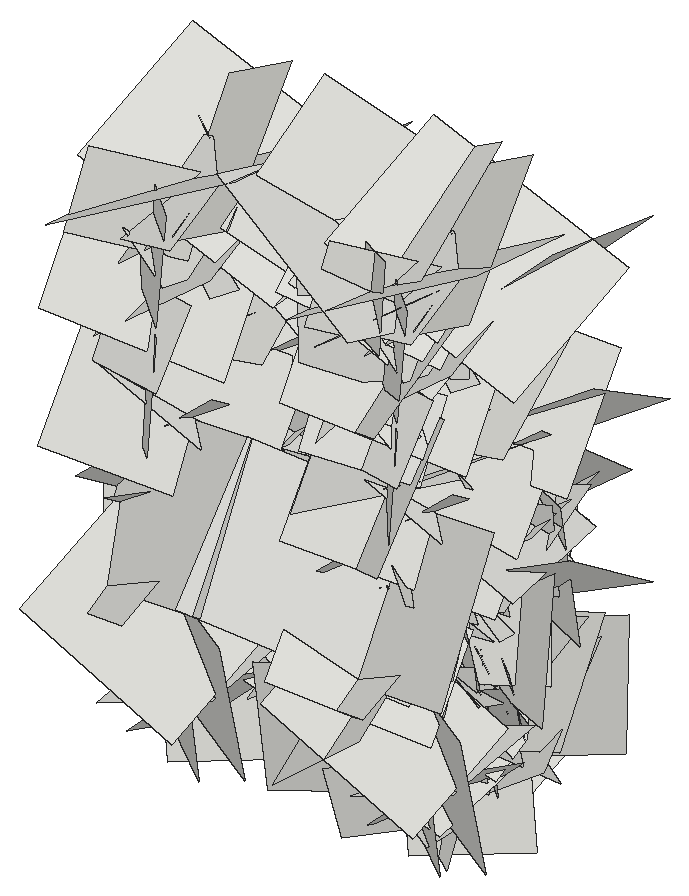
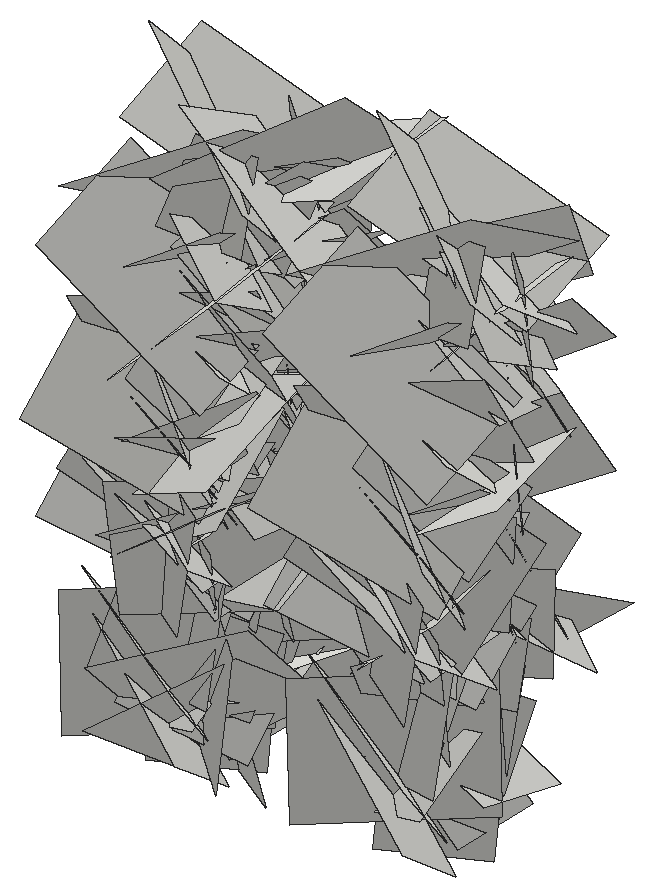
# SketchUp Ruby script. Lengths in inches.
U = 1.inch
M = Sketchup.active_model
def pt(a) = Geom::Point3d.new(a.map { |v| v * U })
def face(e, loops, mat)
  f = e.add_face(loops[0].map { |a| pt(a) })
  loops[1..].each { |l| e.add_face(l.map { |a| pt(a) }).erase! }
  f.material = f.back_material = mat if mat
  f
end
# faces: each face lists its corners as indices into pts; further lists are holes
def faces(e, pts, list, mat = nil) = list.each { |f| face(e, (f[0].is_a?(Array) ? f : [f]).map { |l| l.map { |i| pts[i] } }, mat) }
# xy, xz, yz: faces in a plane at the given z, y or x. An outline is a flat list of corners, or four numbers for a rectangle; further outlines are holes
def ring(l) = l.size == 4 ? [[l[0], l[1]], [l[2], l[1]], [l[2], l[3]], [l[0], l[3]]] : l.each_slice(2).to_a
def flat(e, list, mat, &to3) = list.each { |f| face(e, (f[0].is_a?(Array) ? f : [f]).map { |l| ring(l).map { |u, v| to3.(u, v) } }, mat) }
def xy(e, z, list, mat = nil) = flat(e, list, mat) { |x, y| [x, y, z] }
def xz(e, y, list, mat = nil) = flat(e, list, mat) { |x, z| [x, y, z] }
def yz(e, x, list, mat = nil) = flat(e, list, mat) { |y, z| [x, y, z] }
def lines(e, pts, list) = list.each { |a, b| e.add_line(pt(pts[a]), pt(pts[b])) }
# prism: a flat outline (further loops are holes) pulled along v
def prism(e, loops, v, mat = nil)
  f = face(e, loops, mat); d = Geom::Vector3d.new(v.map { |x| x * U })
  f.pushpull(f.normal.samedirection?(d) ? d.length : -d.length)
end
def box(e, o, s, mat = nil) = prism(e, [[o, [o[0] + s[0], o[1], o[2]], [o[0] + s[0], o[1] + s[1], o[2]], [o[0], o[1] + s[1], o[2]]]], [0, 0, s[2]], mat)
def at(x, y, z, deg = 0) = Geom::Transformation.translation(pt([x, y, z])) * Geom::Transformation.rotation(ORIGIN, Z_AXIS, deg.degrees)
def axes(o, x, y, z) = Geom::Transformation.new([*x, 0, *y, 0, *z, 0, *pt(o).to_a, 1])
def part(name) = M.definitions.add(name)
# library, detail: a bought-in or finely detailed component or shape, given as its bounding box
def library(name, o, s) = part(name).tap { |d| box(d.entities, o, s) }
def detail(e, o, s) = box(e.add_group.entities, o, s)
def put(e, d, t, mat = nil) = e.add_instance(d, t).tap { |i| i.material = mat if mat }
def group(e, t, mat = nil) = e.add_group.tap { |g| g.transformation = t; g.material = mat if mat }.entities
root = M.entities
c1 = part("Component\#6")
p = [[0.01,0,0],[0,3.24,4.54],[4.32,3.24,4.54],[4.33,0,0]]
faces(c1.entities,p,[[0,1,2,3]])
put(root,c1,axes([410.71,170.9375,7.01],[0.11124,0.9843,0.53665],[-0.15751,0.54645,-0.97322],[1.17787,-0.01989,-0.18083]))
put(root,c1,axes([424.49,170.9375,7.01],[-0.11124,0.9843,0.53665],[0.15751,0.54645,-0.97322],[-1.17787,-0.01989,-0.18083]))
put(root,c1,axes([420.52,170.9375,7.01],[0.11124,0.9843,0.53665],[-0.15751,0.54645,-0.97322],[1.17787,-0.01989,-0.18083]))
put(root,c1,axes([410.71,177.17,11.87],[0.09089,-0.73345,-1.16692],[0.11565,-1.16189,0.73831],[1.45639,0.13804,0.0142]))
put(root,c1,axes([424.49,177.17,11.87],[-0.09089,-0.73345,-1.16692],[-0.11565,-1.16189,0.73831],[-1.45639,0.13804,0.0142]))
put(root,c1,axes([420.52,177.17,11.87],[0.09089,-0.73345,-1.16692],[0.11565,-1.16189,0.73831],[1.45639,0.13804,0.0142]))
put(root,c1,axes([414.68,171.15,7.72],[0.19789,0.75168,0.59634],[-0.00491,0.60823,-0.76521],[-1.01706,0.14332,0.11972]))
put(root,c1,axes([420.52,171.15,7.72],[-0.19789,0.75168,0.59634],[0.00491,0.60823,-0.76521],[1.01706,0.14332,0.11972]))
put(root,c1,axes([424.49,171.15,7.72],[0.19789,0.75168,0.59634],[-0.00491,0.60823,-0.76521],[-1.01706,0.14332,0.11972]))
put(root,c1,axes([414.68,175.79,22.11],[-0.09057,-0.18477,-0.67682],[0.07729,-0.68047,0.17656],[-0.73966,-0.04848,0.10132]))
put(root,c1,axes([420.52,175.79,22.11],[0.09057,-0.18477,-0.67682],[-0.07729,-0.68047,0.17656],[0.73966,-0.04848,0.10132]))
put(root,c1,axes([424.49,175.79,22.11],[-0.09057,-0.18477,-0.67682],[0.07729,-0.68047,0.17656],[-0.73966,-0.04848,0.10132]))
put(root,c1,axes([414.68,172.87,15.39],[0.04258,0.36909,0.59744],[-0.18529,0.58484,-0.34955],[-0.72096,-0.1285,0.12512]))
put(root,c1,axes([420.52,172.87,15.39],[-0.04258,0.36909,0.59744],[0.18529,0.58484,-0.34955],[0.72096,-0.1285,0.12512]))
put(root,c1,axes([424.49,172.87,15.39],[0.04258,0.36909,0.59744],[-0.18529,0.58484,-0.34955],[-0.72096,-0.1285,0.12512]))
put(root,c1,axes([410.71,176.71,20],[0.1716,-1.2405,0.25629],[0.15029,0.2745,1.23906],[1.33426,0.12862,-0.17253]))
put(root,c1,axes([424.49,176.71,20],[-0.1716,-1.2405,0.25629],[-0.15029,0.2745,1.23906],[-1.33426,0.12862,-0.17253]))
put(root,c1,axes([420.52,176.71,20],[0.1716,-1.2405,0.25629],[0.15029,0.2745,1.23906],[1.33426,0.12862,-0.17253]))
put(root,c1,axes([414.68,172.9,17.79],[0.05847,0.04666,0.93522],[0.13105,0.92828,-0.05361],[-0.98388,0.12642,0.04844]))
put(root,c1,axes([420.52,172.9,17.79],[-0.05847,0.04666,0.93522],[-0.13105,0.92828,-0.05361],[0.98388,0.12642,0.04844]))
put(root,c1,axes([424.49,172.9,17.79],[0.05847,0.04666,0.93522],[0.13105,0.92828,-0.05361],[-0.98388,0.12642,0.04844]))
put(root,c1,axes([414.68,172.44,13.26],[-0.14239,0.27787,0.83247],[0.25689,0.82117,-0.23499],[-0.89411,0.19168,-0.20009]))
put(root,c1,axes([420.52,172.44,13.26],[0.14239,0.27787,0.83247],[-0.25689,0.82117,-0.23499],[0.89411,0.19168,-0.20009]))
put(root,c1,axes([424.49,172.44,13.26],[-0.14239,0.27787,0.83247],[0.25689,0.82117,-0.23499],[-0.89411,0.19168,-0.20009]))
put(root,c1,axes([414.68,178.76,18.36],[0.19902,-0.79911,-0.76231],[0.1591,-0.74761,0.82067],[-1.1598,-0.23968,-0.01823]))
put(root,c1,axes([420.52,178.76,18.36],[-0.19902,-0.79911,-0.76231],[-0.1591,-0.74761,0.82067],[1.1598,-0.23968,-0.01823]))
put(root,c1,axes([424.49,178.76,18.36],[0.19902,-0.79911,-0.76231],[0.1591,-0.74761,0.82067],[-1.1598,-0.23968,-0.01823]))
put(root,c1,axes([410.71,178.02,21.625],[-0.10055,-0.80704,-0.57155],[0.14009,-0.57937,0.79615],[1.03886,0.00001,-0.16268]))
put(root,c1,axes([424.49,178.02,21.625],[0.10055,-0.80704,-0.57155],[-0.14009,-0.57937,0.79615],[-1.03886,0.00001,-0.16268]))
put(root,c1,axes([420.52,178.02,21.625],[-0.10055,-0.80704,-0.57155],[0.14009,-0.57937,0.79615],[1.03886,0.00001,-0.16268]))
put(root,c1,axes([410.71,171.875,12.53],[-0.03767,0.74177,1.03266],[-0.14299,1.02503,-0.74093],[1.34014,0.13022,-0.05004]))
put(root,c1,axes([424.49,171.875,12.53],[0.03767,0.74177,1.03266],[0.14299,1.02503,-0.74093],[-1.34014,0.13022,-0.05004]))
put(root,c1,axes([420.52,171.875,12.53],[-0.03767,0.74177,1.03266],[-0.14299,1.02503,-0.74093],[1.34014,0.13022,-0.05004]))
put(root,c1,axes([414.68,176.92,18.36],[-0.03591,-0.7978,0.13647],[0.05211,0.13431,0.79737],[-0.85636,0.04162,0.0428]))
put(root,c1,axes([420.52,176.92,18.36],[0.03591,-0.7978,0.13647],[-0.05211,0.13431,0.79737],[0.85636,0.04162,0.0428]))
put(root,c1,axes([424.49,176.92,18.36],[-0.03591,-0.7978,0.13647],[0.05211,0.13431,0.79737],[-0.85636,0.04162,0.0428]))
put(root,c1,axes([410.71,176.79,7.17],[0.05072,0.23896,-1.1979],[0.10512,-1.19562,-0.23454],[1.29052,0.088,0.06618]))
put(root,c1,axes([424.49,176.79,7.17],[-0.05072,0.23896,-1.1979],[-0.10512,-1.19562,-0.23454],[-1.29052,0.088,0.06618]))
put(root,c1,axes([420.52,176.79,7.17],[0.05072,0.23896,-1.1979],[0.10512,-1.19562,-0.23454],[1.29052,0.088,0.06618]))
put(root,c1,axes([414.68,175.07,0.3],[0.05353,-0.16234,0.63718],[0.01427,0.63917,0.16178],[-0.69684,0.00062,0.05226]))
put(root,c1,axes([420.52,175.07,0.3],[-0.05353,-0.16234,0.63718],[-0.01427,0.63917,0.16178],[0.69684,0.00062,0.05226]))
put(root,c1,axes([424.49,175.07,0.3],[0.05353,-0.16234,0.63718],[0.01427,0.63917,0.16178],[-0.69684,0.00062,0.05226]))
put(root,c1,axes([410.71,178.16,17.01],[0.17232,-1.0163,-0.23365],[-0.0611,-0.24487,1.02499],[1.10369,0.14512,0.09322]))
put(root,c1,axes([424.49,178.16,17.01],[-0.17232,-1.0163,-0.23365],[0.0611,-0.24487,1.02499],[-1.10369,0.14512,0.09322]))
put(root,c1,axes([420.52,178.16,17.01],[0.17232,-1.0163,-0.23365],[-0.0611,-0.24487,1.02499],[1.10369,0.14512,0.09322]))
put(root,c1,axes([410.71,178.75,19.8],[0.0392,-0.90326,-0.49419],[-0.16181,-0.49385,0.89122],[1.07932,-0.04123,0.15156]))
put(root,c1,axes([424.49,178.75,19.8],[-0.0392,-0.90326,-0.49419],[0.16181,-0.49385,0.89122],[-1.07932,-0.04123,0.15156]))
put(root,c1,axes([420.52,178.75,19.8],[0.0392,-0.90326,-0.49419],[-0.16181,-0.49385,0.89122],[1.07932,-0.04123,0.15156]))
put(root,c1,axes([414.68,174.43,8.39],[0.03188,0.26889,0.69876],[-0.00311,0.69936,-0.269],[-0.79363,0.00806,0.02912]))
put(root,c1,axes([420.52,174.43,8.39],[-0.03188,0.26889,0.69876],[0.00311,0.69936,-0.269],[0.79363,0.00806,0.02912]))
put(root,c1,axes([424.49,174.43,8.39],[0.03188,0.26889,0.69876],[-0.00311,0.69936,-0.269],[-0.79363,0.00806,0.02912]))
put(root,c1,axes([410.71,179.79,22.45],[0.18749,-0.99323,-0.93091],[-0.09936,-0.94539,0.99088],[1.43954,0.06411,0.18963]))
put(root,c1,axes([424.49,179.79,22.45],[-0.18749,-0.99323,-0.93091],[0.09936,-0.94539,0.99088],[-1.43954,0.06411,0.18963]))
put(root,c1,axes([420.52,179.79,22.45],[0.18749,-0.99323,-0.93091],[-0.09936,-0.94539,0.99088],[1.43954,0.06411,0.18963]))
put(root,c1,axes([410.71,177.03,8.61],[0.03763,-0.79919,0.49947],[-0.19388,0.48448,0.78821],[0.97999,0.12653,0.13676]))
put(root,c1,axes([424.49,177.03,8.61],[-0.03763,-0.79919,0.49947],[0.19388,0.48448,0.78821],[-0.97999,0.12653,0.13676]))
put(root,c1,axes([420.52,177.03,8.61],[0.03763,-0.79919,0.49947],[-0.19388,0.48448,0.78821],[0.97999,0.12653,0.13676]))
put(root,c1,axes([414.68,177.03,9.04],[0.05145,-0.49737,0.47013],[-0.11624,0.45957,0.49752],[-0.71609,-0.11034,-0.04698]))
put(root,c1,axes([420.52,177.03,9.04],[-0.05145,-0.49737,0.47013],[0.11624,0.45957,0.49752],[0.71609,-0.11034,-0.04698]))
put(root,c1,axes([424.49,177.03,9.04],[0.05145,-0.49737,0.47013],[-0.11624,0.45957,0.49752],[-0.71609,-0.11034,-0.04698]))
put(root,c1,axes([410.71,179.02,2.63],[-0.02304,-0.93672,-0.18796],[0.20199,-0.18848,0.91728],[0.99236,0.01662,-0.19107]))
put(root,c1,axes([424.49,179.02,2.63],[0.02304,-0.93672,-0.18796],[-0.20199,-0.18848,0.91728],[-0.99236,0.01662,-0.19107]))
put(root,c1,axes([420.52,179.02,2.63],[-0.02304,-0.93672,-0.18796],[0.20199,-0.18848,0.91728],[0.99236,0.01662,-0.19107]))
put(root,c1,axes([414.68,175.31,3.87],[0.17194,0.72285,-0.14796],[0.1038,-0.17124,-0.72925],[-0.77519,0.1374,-0.13047]))
put(root,c1,axes([420.52,175.31,3.87],[-0.17194,0.72285,-0.14796],[-0.1038,-0.17124,-0.72925],[0.77519,0.1374,-0.13047]))
put(root,c1,axes([424.49,175.31,3.87],[0.17194,0.72285,-0.14796],[0.1038,-0.17124,-0.72925],[-0.77519,0.1374,-0.13047]))
put(root,c1,axes([410.71,173.88,22.27],[0.13701,1.18016,0.66561],[0.07419,0.66193,-1.18721],[1.4343,-0.14697,-0.00217]))
put(root,c1,axes([424.49,173.88,22.27],[-0.13701,1.18016,0.66561],[-0.07419,0.66193,-1.18721],[-1.4343,-0.14697,-0.00217]))
put(root,c1,axes([420.52,173.88,22.27],[0.13701,1.18016,0.66561],[0.07419,0.66193,-1.18721],[1.4343,-0.14697,-0.00217]))
put(root,c1,axes([410.71,175.28,5.97],[-0.1544,0.17587,1.10387],[0.02973,1.11343,-0.17369],[1.18449,-0.00502,0.14825]))
put(root,c1,axes([424.49,175.28,5.97],[0.1544,0.17587,1.10387],[-0.02973,1.11343,-0.17369],[-1.18449,-0.00502,0.14825]))
put(root,c1,axes([420.52,175.28,5.97],[-0.1544,0.17587,1.10387],[0.02973,1.11343,-0.17369],[1.18449,-0.00502,0.14825]))
put(root,c1,axes([410.71,174.05,15.13],[-0.29087,1.34123,-0.04275],[0.1118,-0.02194,-1.36543],[1.41802,0.27684,0.09888]))
put(root,c1,axes([424.49,174.05,15.13],[0.29087,1.34123,-0.04275],[-0.1118,-0.02194,-1.36543],[-1.41802,0.27684,0.09888]))
put(root,c1,axes([420.52,174.05,15.13],[-0.29087,1.34123,-0.04275],[0.1118,-0.02194,-1.36543],[1.41802,0.27684,0.09888]))
put(root,c1,axes([410.71,177.91,2.6],[0.0759,-0.493,0.60539],[0.11612,0.60826,0.48238],[0.8194,-0.04053,-0.12444]))
put(root,c1,axes([424.49,177.91,2.6],[-0.0759,-0.493,0.60539],[-0.11612,0.60826,0.48238],[-0.8194,-0.04053,-0.12444]))
put(root,c1,axes([420.52,177.91,2.6],[0.0759,-0.493,0.60539],[0.11612,0.60826,0.48238],[0.8194,-0.04053,-0.12444]))
put(root,c1,axes([414.68,179.07,16.9375],[-0.01654,-0.76992,0.15337],[0.18248,0.14631,0.752],[-0.8119,0.04857,0.16589]))
put(root,c1,axes([420.52,179.07,16.9375],[0.01654,-0.76992,0.15337],[-0.18248,0.14631,0.752],[0.8119,0.04857,0.16589]))
put(root,c1,axes([424.49,179.07,16.9375],[-0.01654,-0.76992,0.15337],[0.18248,0.14631,0.752],[-0.8119,0.04857,0.16589]))
put(root,c1,axes([410.71,177.25,5.58],[0.00826,-0.19404,0.73725],[0.12542,0.72866,0.19053],[0.79831,-0.11247,-0.03756]))
put(root,c1,axes([424.49,177.25,5.58],[-0.00826,-0.19404,0.73725],[-0.12542,0.72866,0.19053],[-0.79831,-0.11247,-0.03756]))
put(root,c1,axes([420.52,177.25,5.58],[0.00826,-0.19404,0.73725],[0.12542,0.72866,0.19053],[0.79831,-0.11247,-0.03756]))
put(root,c1,axes([414.68,178.9,4.98],[0.12785,-0.58421,0.25103],[-0.01096,0.25367,0.59532],[-0.67392,-0.11496,0.03794]))
put(root,c1,axes([420.52,178.9,4.98],[-0.12785,-0.58421,0.25103],[0.01096,0.25367,0.59532],[0.67392,-0.11496,0.03794]))
put(root,c1,axes([424.49,178.9,4.98],[0.12785,-0.58421,0.25103],[-0.01096,0.25367,0.59532],[-0.67392,-0.11496,0.03794]))
put(root,c1,axes([414.68,177.55,19],[0.11507,-0.3549,0.71119],[0.00206,0.71791,0.35796],[-0.84251,-0.04671,0.09801]))
put(root,c1,axes([420.52,177.55,19],[-0.11507,-0.3549,0.71119],[-0.00206,0.71791,0.35796],[0.84251,-0.04671,0.09801]))
put(root,c1,axes([424.49,177.55,19],[0.11507,-0.3549,0.71119],[0.00206,0.71791,0.35796],[-0.84251,-0.04671,0.09801]))
put(root,c1,axes([410.71,179.43,6.59],[0.14458,-1.15784,0.73248],[0.20973,0.74503,1.14083],[1.43706,0.00775,-0.24019]))
put(root,c1,axes([424.49,179.43,6.59],[-0.14458,-1.15784,0.73248],[-0.20973,0.74503,1.14083],[-1.43706,0.00775,-0.24019]))
put(root,c1,axes([420.52,179.43,6.59],[0.14458,-1.15784,0.73248],[0.20973,0.74503,1.14083],[1.43706,0.00775,-0.24019]))
put(root,c1,axes([410.71,177.67,8.79],[0.10774,-0.22129,0.90038],[0.20078,0.89162,0.19775],[0.96207,-0.1613,-0.1421]))
put(root,c1,axes([424.49,177.67,8.79],[-0.10774,-0.22129,0.90038],[-0.20078,0.89162,0.19775],[-0.96207,-0.1613,-0.1421]))
put(root,c1,axes([420.52,177.67,8.79],[0.10774,-0.22129,0.90038],[0.20078,0.89162,0.19775],[0.96207,-0.1613,-0.1421]))
put(root,c1,axes([414.68,179.66,2.51],[0.14219,-0.09473,-0.68692],[-0.01318,-0.69988,0.09409],[-0.73491,-0.00578,-0.13459]))
put(root,c1,axes([420.52,179.66,2.51],[-0.14219,-0.09473,-0.68692],[0.01318,-0.69988,0.09409],[0.73491,-0.00578,-0.13459]))
put(root,c1,axes([424.49,179.66,2.51],[0.14219,-0.09473,-0.68692],[-0.01318,-0.69988,0.09409],[-0.73491,-0.00578,-0.13459]))
put(root,c1,axes([414.68,180.59,3.91],[0.10883,-0.74668,-0.23347],[-0.0349,-0.23939,0.75113],[-0.82853,-0.08799,-0.06231]))
put(root,c1,axes([420.52,180.59,3.91],[-0.10883,-0.74668,-0.23347],[0.0349,-0.23939,0.75113],[0.82853,-0.08799,-0.06231]))
put(root,c1,axes([424.49,180.59,3.91],[0.10883,-0.74668,-0.23347],[-0.0349,-0.23939,0.75113],[-0.82853,-0.08799,-0.06231]))
put(root,c1,axes([414.68,180.83,12.7],[0.12371,-0.65209,-0.45157],[0.04757,-0.45027,0.66181],[-0.83942,-0.12162,-0.02905]))
put(root,c1,axes([420.52,180.83,12.7],[-0.12371,-0.65209,-0.45157],[-0.04757,-0.45027,0.66181],[0.83942,-0.12162,-0.02905]))
put(root,c1,axes([424.49,180.83,12.7],[0.12371,-0.65209,-0.45157],[0.04757,-0.45027,0.66181],[-0.83942,-0.12162,-0.02905]))
put(root,c1,axes([410.71,180.99,16.6875],[0.01817,-0.80344,-0.66577],[0.22863,-0.64876,0.78846],[1.08217,0.15055,-0.1554]))
put(root,c1,axes([424.49,180.99,16.6875],[-0.01817,-0.80344,-0.66577],[-0.22863,-0.64876,0.78846],[-1.08217,0.15055,-0.1554]))
put(root,c1,axes([420.52,180.99,16.6875],[0.01817,-0.80344,-0.66577],[0.22863,-0.64876,0.78846],[1.08217,0.15055,-0.1554]))
put(root,c1,axes([410.71,176.29,14.82],[0.00549,0.62123,1.00169],[0.24363,0.98194,-0.61017],[1.22543,-0.19801,0.11682]))
put(root,c1,axes([424.49,176.29,14.82],[-0.00549,0.62123,1.00169],[-0.24363,0.98194,-0.61017],[-1.22543,-0.19801,0.11682]))
put(root,c1,axes([420.52,176.29,14.82],[0.00549,0.62123,1.00169],[0.24363,0.98194,-0.61017],[1.22543,-0.19801,0.11682]))
put(root,c1,axes([414.68,178.54,4.68],[-0.06155,-0.26232,0.60589],[-0.0363,0.6086,0.26022],[-0.69891,-0.00851,-0.06687]))
put(root,c1,axes([420.52,178.54,4.68],[0.06155,-0.26232,0.60589],[0.0363,0.6086,0.26022],[0.69891,-0.00851,-0.06687]))
put(root,c1,axes([424.49,178.54,4.68],[-0.06155,-0.26232,0.60589],[-0.0363,0.6086,0.26022],[-0.69891,-0.00851,-0.06687]))
put(root,c1,axes([424.49,179.8125,11.71],[-0.00414,-0.7832,0.49624],[0.01003,0.49619,0.78318],[-0.98275,0.00836,0.0059]))
put(root,c1,axes([410.71,179.8125,11.71],[0.00414,-0.7832,0.49624],[-0.01003,0.49619,0.78318],[0.98275,0.00836,0.0059]))
put(root,c1,axes([420.52,179.8125,11.71],[0.00414,-0.7832,0.49624],[-0.01003,0.49619,0.78318],[0.98275,0.00836,0.0059]))
put(root,c1,axes([410.71,181.49,10.05],[0.07357,-0.24485,-1.22332],[0.09578,-1.221,0.24951],[1.31896,0.10233,0.05011]))
put(root,c1,axes([424.49,181.49,10.05],[-0.07357,-0.24485,-1.22332],[-0.09578,-1.221,0.24951],[-1.31896,0.10233,0.05011]))
put(root,c1,axes([420.52,181.49,10.05],[0.07357,-0.24485,-1.22332],[0.09578,-1.221,0.24951],[1.31896,0.10233,0.05011]))
put(root,c1,axes([414.68,181.21,19.66],[0.0984,-0.57654,-0.29954],[0.01889,-0.30021,0.58335],[-0.68843,-0.09064,-0.02681]))
put(root,c1,axes([420.52,181.21,19.66],[-0.0984,-0.57654,-0.29954],[-0.01889,-0.30021,0.58335],[0.68843,-0.09064,-0.02681]))
put(root,c1,axes([424.49,181.21,19.66],[0.0984,-0.57654,-0.29954],[0.01889,-0.30021,0.58335],[-0.68843,-0.09064,-0.02681]))
put(root,c1,axes([414.68,181.24,7.39],[0.09835,-0.8461,0.11424],[0.10744,0.12502,0.84359],[-0.89861,-0.07766,0.11336]))
put(root,c1,axes([420.52,181.24,7.39],[-0.09835,-0.8461,0.11424],[-0.10744,0.12502,0.84359],[0.89861,-0.07766,0.11336]))
put(root,c1,axes([424.49,181.24,7.39],[0.09835,-0.8461,0.11424],[0.10744,0.12502,0.84359],[-0.89861,-0.07766,0.11336]))
put(root,c1,axes([410.71,180.26,8.26],[-0.04265,-1.00211,0.75475],[-0.17142,0.75298,0.99114],[1.31872,0.06547,0.15325]))
put(root,c1,axes([424.49,180.26,8.26],[0.04265,-1.00211,0.75475],[0.17142,0.75298,0.99114],[-1.31872,0.06547,0.15325]))
put(root,c1,axes([420.52,180.26,8.26],[-0.04265,-1.00211,0.75475],[-0.17142,0.75298,0.99114],[1.31872,0.06547,0.15325]))
put(root,c1,axes([410.71,182.69,9.96],[-0.0402,-0.96504,-0.67279],[0.04089,-0.67379,0.96431],[1.24632,-0.00902,-0.05333]))
put(root,c1,axes([424.49,182.69,9.96],[0.0402,-0.96504,-0.67279],[-0.04089,-0.67379,0.96431],[-1.24632,-0.00902,-0.05333]))
put(root,c1,axes([420.52,182.69,9.96],[-0.0402,-0.96504,-0.67279],[0.04089,-0.67379,0.96431],[1.24632,-0.00902,-0.05333]))
put(root,c1,axes([410.71,182.3,13.14],[0.06012,-0.59744,-0.78978],[-0.12867,-0.78931,0.58836],[1.0418,-0.06301,0.11824]))
put(root,c1,axes([424.49,182.3,13.14],[-0.06012,-0.59744,-0.78978],[0.12867,-0.78931,0.58836],[-1.0418,-0.06301,0.11824]))
put(root,c1,axes([420.52,182.3,13.14],[0.06012,-0.59744,-0.78978],[-0.12867,-0.78931,0.58836],[1.0418,-0.06301,0.11824]))
put(root,c1,axes([414.68,181.23,7.68],[-0.09173,-0.20092,-0.6203],[0.07215,-0.6251,0.19298],[-0.68737,-0.0388,0.10304]))
put(root,c1,axes([420.52,181.23,7.68],[0.09173,-0.20092,-0.6203],[-0.07215,-0.6251,0.19298],[0.68737,-0.0388,0.10304]))
put(root,c1,axes([424.49,181.23,7.68],[-0.09173,-0.20092,-0.6203],[0.07215,-0.6251,0.19298],[-0.68737,-0.0388,0.10304]))
put(root,c1,axes([410.71,179.12,5.58],[0.07323,0.67973,-0.51678],[0.08286,-0.52133,-0.67526],[0.90131,-0.0073,0.10406]))
put(root,c1,axes([424.49,179.12,5.58],[-0.07323,0.67973,-0.51678],[-0.08286,-0.52133,-0.67526],[-0.90131,-0.0073,0.10406]))
put(root,c1,axes([420.52,179.12,5.58],[0.07323,0.67973,-0.51678],[0.08286,-0.52133,-0.67526],[0.90131,-0.0073,0.10406]))
put(root,c1,axes([410.71,181.89,8.77],[0.15486,-1.04414,-0.08659],[-0.04063,-0.0927,1.0531],[1.10985,0.1423,0.05063]))
put(root,c1,axes([424.49,181.89,8.77],[-0.15486,-1.04414,-0.08659],[0.04063,-0.0927,1.0531],[-1.10985,0.1423,0.05063]))
put(root,c1,axes([420.52,181.89,8.77],[0.15486,-1.04414,-0.08659],[-0.04063,-0.0927,1.0531],[1.10985,0.1423,0.05063]))
put(root,c1,axes([410.71,182.08,15.67],[0.13861,-1.35642,0.31459],[-0.2886,0.28497,1.34186],[1.44748,0.1867,0.23742]))
put(root,c1,axes([424.49,182.08,15.67],[-0.13861,-1.35642,0.31459],[0.2886,0.28497,1.34186],[-1.44748,0.1867,0.23742]))
put(root,c1,axes([420.52,182.08,15.67],[0.13861,-1.35642,0.31459],[-0.2886,0.28497,1.34186],[1.44748,0.1867,0.23742]))
put(root,c1,axes([424.49,180.69,8.55],[0.12889,0.40226,-0.91097],[0.04748,-0.91901,-0.39983],[-1.05451,0.00779,-0.12935]))
put(root,c1,axes([410.71,180.69,8.55],[-0.12889,0.40226,-0.91097],[-0.04748,-0.91901,-0.39983],[1.05451,0.00779,-0.12935]))
put(root,c1,axes([420.52,180.69,8.55],[-0.12889,0.40226,-0.91097],[-0.04748,-0.91901,-0.39983],[1.05451,0.00779,-0.12935]))
put(root,c1,axes([410.71,178.03,1.86],[0.09591,-0.07879,1.2407],[-0.19288,1.22975,0.09137],[1.3036,0.18775,-0.07776]))
put(root,c1,axes([424.49,178.03,1.86],[-0.09591,-0.07879,1.2407],[0.19288,1.22975,0.09137],[-1.3036,0.18775,-0.07776]))
put(root,c1,axes([420.52,178.03,1.86],[0.09591,-0.07879,1.2407],[-0.19288,1.22975,0.09137],[1.3036,0.18775,-0.07776]))
put(root,c1,axes([414.68,178.57,11.38],[0.09025,0.42259,0.64735],[-0.15778,0.64804,-0.40347],[-0.80413,-0.07973,0.15182]))
put(root,c1,axes([420.52,178.57,11.38],[-0.09025,0.42259,0.64735],[0.15778,0.64804,-0.40347],[0.80413,-0.07973,0.15182]))
put(root,c1,axes([424.49,178.57,11.38],[0.09025,0.42259,0.64735],[-0.15778,0.64804,-0.40347],[-0.80413,-0.07973,0.15182]))
put(root,c1,axes([410.71,181.48,10.98],[0.16941,-1.10786,0.62997],[-0.04307,0.63015,1.11849],[1.35023,0.1591,-0.04336]))
put(root,c1,axes([424.49,181.48,10.98],[-0.16941,-1.10786,0.62997],[0.04307,0.63015,1.11849],[-1.35023,0.1591,-0.04336]))
put(root,c1,axes([420.52,181.48,10.98],[0.16941,-1.10786,0.62997],[-0.04307,0.63015,1.11849],[1.35023,0.1591,-0.04336]))
put(root,c1,axes([410.71,183.39,2.71],[0.21072,-0.93049,-0.66529],[-0.0846,-0.6849,0.93407],[1.20954,0.1142,0.18123]))
put(root,c1,axes([424.49,183.39,2.71],[-0.21072,-0.93049,-0.66529],[0.0846,-0.6849,0.93407],[-1.20954,0.1142,0.18123]))
put(root,c1,axes([420.52,183.39,2.71],[0.21072,-0.93049,-0.66529],[-0.0846,-0.6849,0.93407],[1.20954,0.1142,0.18123]))
put(root,c1,axes([410.71,182.3,11.84],[0.17648,0.01407,-1.1199],[0.09677,-1.12861,-0.00061],[1.18323,0.09021,0.16708]))
put(root,c1,axes([424.49,182.3,11.84],[-0.17648,0.01407,-1.1199],[-0.09677,-1.12861,-0.00061],[-1.18323,0.09021,0.16708]))
put(root,c1,axes([420.52,182.3,11.84],[0.17648,0.01407,-1.1199],[0.09677,-1.12861,-0.00061],[1.18323,0.09021,0.16708]))
put(root,c1,axes([410.71,183.3125,5.12],[0.15127,-0.71846,-0.81538],[0.11003,-0.80961,0.73154],[1.14669,0.17246,0.03737]))
put(root,c1,axes([424.49,183.3125,5.12],[-0.15127,-0.71846,-0.81538],[-0.11003,-0.80961,0.73154],[-1.14669,0.17246,0.03737]))
put(root,c1,axes([420.52,183.3125,5.12],[0.15127,-0.71846,-0.81538],[0.11003,-0.80961,0.73154],[1.14669,0.17246,0.03737]))
